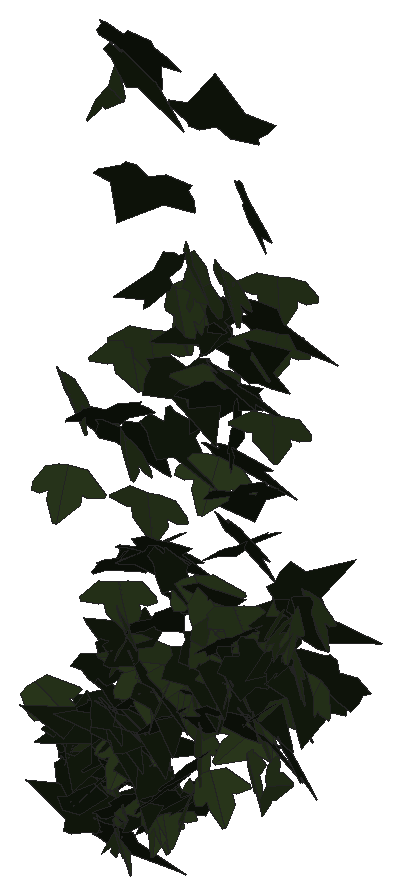
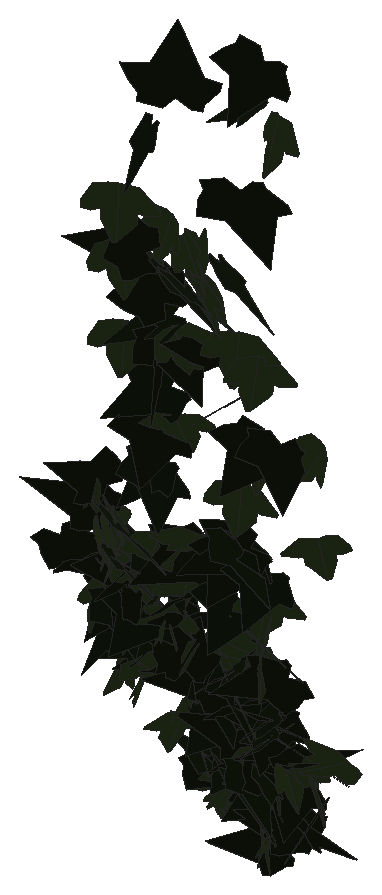
# SketchUp Ruby script. Lengths in inches.
U = 1.inch
M = Sketchup.active_model
def pt(a) = Geom::Point3d.new(a.map { |v| v * U })
def face(e, loops, mat)
  f = e.add_face(loops[0].map { |a| pt(a) })
  loops[1..].each { |l| e.add_face(l.map { |a| pt(a) }).erase! }
  f.material = f.back_material = mat if mat
  f
end
# faces: each face lists its corners as indices into pts; further lists are holes
def faces(e, pts, list, mat = nil) = list.each { |f| face(e, (f[0].is_a?(Array) ? f : [f]).map { |l| l.map { |i| pts[i] } }, mat) }
# xy, xz, yz: faces in a plane at the given z, y or x. An outline is a flat list of corners, or four numbers for a rectangle; further outlines are holes
def ring(l) = l.size == 4 ? [[l[0], l[1]], [l[2], l[1]], [l[2], l[3]], [l[0], l[3]]] : l.each_slice(2).to_a
def flat(e, list, mat, &to3) = list.each { |f| face(e, (f[0].is_a?(Array) ? f : [f]).map { |l| ring(l).map { |u, v| to3.(u, v) } }, mat) }
def xy(e, z, list, mat = nil) = flat(e, list, mat) { |x, y| [x, y, z] }
def xz(e, y, list, mat = nil) = flat(e, list, mat) { |x, z| [x, y, z] }
def yz(e, x, list, mat = nil) = flat(e, list, mat) { |y, z| [x, y, z] }
def lines(e, pts, list) = list.each { |a, b| e.add_line(pt(pts[a]), pt(pts[b])) }
# prism: a flat outline (further loops are holes) pulled along v
def prism(e, loops, v, mat = nil)
  f = face(e, loops, mat); d = Geom::Vector3d.new(v.map { |x| x * U })
  f.pushpull(f.normal.samedirection?(d) ? d.length : -d.length)
end
def box(e, o, s, mat = nil) = prism(e, [[o, [o[0] + s[0], o[1], o[2]], [o[0] + s[0], o[1] + s[1], o[2]], [o[0], o[1] + s[1], o[2]]]], [0, 0, s[2]], mat)
def at(x, y, z, deg = 0) = Geom::Transformation.translation(pt([x, y, z])) * Geom::Transformation.rotation(ORIGIN, Z_AXIS, deg.degrees)
def axes(o, x, y, z) = Geom::Transformation.new([*x, 0, *y, 0, *z, 0, *pt(o).to_a, 1])
def part(name) = M.definitions.add(name)
# library, detail: a bought-in or finely detailed component or shape, given as its bounding box
def library(name, o, s) = part(name).tap { |d| box(d.entities, o, s) }
def detail(e, o, s) = box(e.add_group.entities, o, s)
def put(e, d, t, mat = nil) = e.add_instance(d, t).tap { |i| i.material = mat if mat }
def group(e, t, mat = nil) = e.add_group.tap { |g| g.transformation = t; g.material = mat if mat }.entities
root = M.entities
M.materials.add("1026 AP 7946 SUNNY SIDE UP").color = [254, 231, 186]
M.materials.add("efeu1").color = [18, 25, 13]
M.materials.add("efeu2").color = [43, 57, 29]
c1 = part("ivyleaf_10")
p = [[0,0.5,-0.03],[-0.0625,2.02,-0.43],[-0.19,2.01,-0.46],[-0.54,1.05,-0.29],[-0.52,0.625,-0.18],[-0.83,0.76,-0.28],
  [-1.16,0.64,-0.33],[-1.15,0.33,-0.24],[-0.77,-0.39,0.02],[-0.3,-0.51,0.16],[0.04,-0.48,0.23],[-0.02,2.01,-0.4375],
  [-0.06,2.01,-0.43],[0.04,-0.49,0.23],[0.67,-0.49,0.14],[1.38,0.36,-0.2],[1.375,0.51,-0.24],[0.81,0.65,-0.19],
  [0.62,0.59,-0.15],[0.6,1.09,-0.28],[0.5,1.23,-0.31]]
faces(c1.entities,p,[[0,1,2,3,4,5,6,7,8,9,10],[11,12,0,13,14,15,16,17,18,19,20]],"efeu2")
c2 = part("ivyleaf_9")
p = [[1.54,2.16,1.25],[1.36,2.04,1.19],[-0.21,0.99,0.68],[-0.71,1.11,0.82],[-0.85,0.86,0.67],[-0.8,0.17,0.21],
  [-0.9,-0.01,0.1],[-0.67,-0.16,-0.02],[-0.08,-0.08,-0.05],[-0.03,-0.6,-0.4],[0.65,-0.88,-0.66],[0.83,-0.6,-0.49],
  [1.29,-0.42,-0.43],[1.8125,-0.07,-0.26],[1.21,0.44,0.15]]
faces(c2.entities,p,[[0,1,2,3,4,5,6,7,8,9,10,11,12,13,14]],"efeu1")
put(root,c1,axes([118.09,212.91,269.5],[0.24792,0.07326,0.21006],[0.30683,0.06038,-0.17781],[-0.14662,0.25024,-0.01692]),"1026 AP 7946 SUNNY SIDE UP")
put(root,c1,axes([118.42,212.92,272.64],[0.29256,0.20397,-0.05662],[-0.07089,-0.03479,-0.28445],[-0.325,0.1912,0.01108]),"1026 AP 7946 SUNNY SIDE UP")
put(root,c2,axes([118.43,212.86,268.69],[0.20932,-0.05573,-0.25304],[-0.25797,0.19116,-0.13534],[0.29986,0.20336,0.0602]),"1026 AP 7946 SUNNY SIDE UP")
put(root,c1,axes([118.49,212.93,269.02],[0.21124,-0.22763,0.00822],[0.0214,-0.00272,-0.2721],[0.35758,0.13463,0.01143]),"1026 AP 7946 SUNNY SIDE UP")
put(root,c1,axes([118.46,212.92,273.98],[-0.295,0.19309,-0.09552],[0.08489,-0.07815,-0.27738],[-0.3267,-0.19466,0.01417]),"1026 AP 7946 SUNNY SIDE UP")
put(root,c2,axes([118.87,212.95,269.2],[-0.11732,0.02044,0.26005],[-0.37111,-0.10071,-0.06409],[0.1439,-0.24307,0.04674]),"1026 AP 7946 SUNNY SIDE UP")
put(root,c2,axes([118.98,212.75,268.2],[-0.19293,0.10643,0.21232],[-0.26123,0.12141,-0.16626],[-0.25332,-0.20626,0.00975]),"1026 AP 7946 SUNNY SIDE UP")
put(root,c2,axes([118.83,212.96,269.2],[-0.26754,-0.19874,-0.02254],[0.04761,0.0013,-0.26856],[0.31058,-0.1714,0.02175]),"1026 AP 7946 SUNNY SIDE UP")
put(root,c2,axes([119.08,212.88,269.46],[-0.39718,0.08165,0.02283],[-0.0584,-0.04588,-0.26784],[-0.11933,-0.24934,0.05509]),"1026 AP 7946 SUNNY SIDE UP")
put(root,c1,axes([118.9,212.99,269.16],[-0.03146,-0.26053,0.00592],[-0.00776,-0.00687,-0.26918],[0.40974,-0.02013,-0.00465]),"1026 AP 7946 SUNNY SIDE UP")
put(root,c1,axes([118.8125,212.92,269.17],[0.38091,0.09128,-0.0266],[-0.02164,-0.03767,-0.26509],[-0.14782,0.24075,-0.02975]),"1026 AP 7946 SUNNY SIDE UP")
put(root,c2,axes([118.92,212.81,268.875],[0.31785,0.10905,-0.12331],[-0.17985,-0.04075,-0.23626],[-0.18124,0.23168,0.01818]),"1026 AP 7946 SUNNY SIDE UP")
put(root,c2,axes([119.09,212.88,273.84],[0.16247,0.25998,-0.05975],[-0.05027,-0.05124,-0.2883],[-0.41633,0.10764,0.0115]),"1026 AP 7946 SUNNY SIDE UP")
put(root,c2,axes([118.83,212.76,268.13],[0.11077,0.02216,0.27527],[0.41323,0.04838,-0.07526],[-0.08254,0.27194,-0.00739]),"1026 AP 7946 SUNNY SIDE UP")
put(root,c2,axes([119.18,212.98,268.8125],[0.16812,0.08963,0.22693],[-0.29764,-0.11321,0.14178],[0.22514,-0.21659,0.01797]),"1026 AP 7946 SUNNY SIDE UP")
put(root,c1,axes([119.22,212.76,278.48],[-0.04949,-0.23028,-0.236],[0.03438,0.22681,-0.23802],[0.50813,-0.03777,-0.00688]),"1026 AP 7946 SUNNY SIDE UP")
put(root,c2,axes([119.32,212.96,269.03],[-0.24075,0.12645,-0.17342],[0.14335,-0.14876,-0.20056],[-0.29942,-0.1729,0.04342]),"1026 AP 7946 SUNNY SIDE UP")
put(root,c1,axes([119.31,212.88,268.05],[0.04735,-0.25138,-0.07093],[0.00458,0.06819,-0.26019],[0.40921,0.02832,0.01112]),"1026 AP 7946 SUNNY SIDE UP")
put(root,c2,axes([119.61,212.84,269.59],[-0.30837,0.0886,0.15521],[-0.25586,-0.01186,-0.2118],[-0.09845,-0.24671,0.06429]),"1026 AP 7946 SUNNY SIDE UP")
put(root,c2,axes([119.29,212.77,269.75],[0.31651,0.16304,-0.08841],[-0.10827,-0.0528,-0.26716],[-0.26945,0.21273,0.0035]),"1026 AP 7946 SUNNY SIDE UP")
put(root,c2,axes([119.06,212.84,270.4],[0.0328,0.02519,-0.28105],[0.15959,0.25357,0.03358],[0.40038,-0.10314,0.00964]),"1026 AP 7946 SUNNY SIDE UP")
put(root,c1,axes([119.06,212.96,268.48],[0.05343,-0.00684,0.26484],[0.34112,-0.13856,-0.03414],[0.21726,0.21923,-0.01152]),"1026 AP 7946 SUNNY SIDE UP")
put(root,c2,axes([119.32,212.88,271.85],[0.18106,0.24801,0.05859],[0.04737,0.04714,-0.28132],[-0.39679,0.1188,-0.00685]),"1026 AP 7946 SUNNY SIDE UP")
put(root,c1,axes([119.3,212.87,268],[-0.12273,0.24977,-0.00755],[-0.00135,-0.00943,-0.26962],[-0.39298,-0.07797,0.00328]),"1026 AP 7946 SUNNY SIDE UP")
put(root,c1,axes([119.35,212.9,270.61],[0.05879,-0.24298,-0.1247],[0.03435,0.12311,-0.24977],[0.42449,0.02369,0.03748]),"1026 AP 7946 SUNNY SIDE UP")
put(root,c1,axes([119.4,212.82,271.06],[-0.25214,0.21535,0.07726],[-0.08709,0.05062,-0.27595],[-0.34718,-0.1691,0.01311]),"1026 AP 7946 SUNNY SIDE UP")
put(root,c2,axes([119.21,212.96,269.49],[0.04065,-0.26337,-0.00088],[-0.00091,-0.0007,-0.27263],[0.41412,0.02585,-0.00051]),"1026 AP 7946 SUNNY SIDE UP")
put(root,c2,axes([119.21,212.89,269.75],[0.07815,-0.25739,-0.06364],[-0.01244,0.0599,-0.26968],[0.41549,0.05021,0.00389]),"1026 AP 7946 SUNNY SIDE UP")
put(root,c2,axes([119.67,212.74,270.77],[-0.15701,0.19537,0.17804],[-0.20314,0.12239,-0.22013],[-0.35498,-0.15645,0.04722]),"1026 AP 7946 SUNNY SIDE UP")
put(root,c1,axes([119.37,212.8125,271.43],[-0.33033,-0.17867,-0.03595],[0.10202,-0.02528,-0.27726],[0.26713,-0.21129,0.06143]),"1026 AP 7946 SUNNY SIDE UP")
put(root,c2,axes([119.14,212.92,269.89],[0.28724,-0.19735,0.0034],[0.03742,0.01604,-0.2754],[0.30812,0.18203,0.03028]),"1026 AP 7946 SUNNY SIDE UP")
put(root,c2,axes([119.56,212.97,268.88],[-0.0665,0.25692,-0.02253],[-0.00284,-0.02393,-0.26832],[-0.40563,-0.04195,0.00557]),"1026 AP 7946 SUNNY SIDE UP")
put(root,c2,axes([119.1,212.88,267.89],[0.32602,-0.0627,0.1501],[0.22377,-0.0337,-0.22322],[0.11133,0.25137,0.0091]),"1026 AP 7946 SUNNY SIDE UP")
put(root,c1,axes([119.43,212.87,269.22],[0.2623,0.18245,-0.10579],[-0.08951,-0.0882,-0.25465],[-0.31764,0.17552,-0.0156]),"1026 AP 7946 SUNNY SIDE UP")
put(root,c2,axes([119.19,212.92,269.67],[0.29189,-0.19266,0.01676],[0.04788,0.00535,-0.27433],[0.30038,0.18636,0.02745]),"1026 AP 7946 SUNNY SIDE UP")
put(root,c1,axes([119.55,212.75,273.58],[-0.35382,0.16193,0.07425],[-0.10708,0.02695,-0.28488],[-0.25667,-0.23446,0.01649]),"1026 AP 7946 SUNNY SIDE UP")
put(root,c1,axes([119.5,212.86,274.85],[-0.31078,-0.20935,-0.03393],[0.08942,-0.01066,-0.29244],[0.32071,-0.19989,0.04867]),"1026 AP 7946 SUNNY SIDE UP")
put(root,c2,axes([119.41,212.64,268.5],[0.22845,0.15593,0.15554],[0.14414,0.11943,-0.21853],[-0.30828,0.17139,0.01309]),"1026 AP 7946 SUNNY SIDE UP")
put(root,c2,axes([119.43,212.81,273.72],[0.42519,0.10335,-0.02983],[-0.02856,-0.03489,-0.29723],[-0.16658,0.26977,-0.02518]),"1026 AP 7946 SUNNY SIDE UP")
put(root,c2,axes([119.53,212.72,279.31],[0.45636,0.04275,-0.11429],[-0.17147,-0.02247,-0.30229],[-0.07537,0.30998,-0.0043]),"1026 AP 7946 SUNNY SIDE UP")
put(root,c2,axes([119.9,212.8,268.61],[-0.18903,0.26611,0.12825],[-0.09243,0.10834,-0.30006],[-0.45159,-0.13357,0.00773]),"1026 AP 7946 SUNNY SIDE UP")
put(root,c2,axes([119.83,212.9,272.18],[-0.06925,0.27367,-0.03072],[-0.07828,-0.03916,-0.28011],[-0.42601,-0.03729,0.05647]),"1026 AP 7946 SUNNY SIDE UP")
put(root,c2,axes([119.77,212.84,277.35],[0.23768,0.16312,-0.23088],[-0.21813,-0.1777,-0.22973],[-0.3787,0.20473,-0.01258]),"1026 AP 7946 SUNNY SIDE UP")
put(root,c2,axes([119.39,212.88,278.92],[0.28834,-0.24691,-0.04076],[0.0088,0.05139,-0.3145],[0.39276,0.18012,0.03697]),"1026 AP 7946 SUNNY SIDE UP")
put(root,c1,axes([119.72,212.93,269.875],[0.1918,-0.23196,0.03149],[0.00627,-0.03389,-0.2699],[0.36811,0.12144,-0.01181]),"1026 AP 7946 SUNNY SIDE UP")
put(root,c2,axes([119.81,212.8,270.13],[0.05112,0.26282,-0.04436],[-0.00292,-0.04466,-0.27306],[-0.41915,0.03236,-0.00351]),"1026 AP 7946 SUNNY SIDE UP")
put(root,c1,axes([120.06,212.84,270.62],[0.15195,-0.01841,-0.31053],[-0.47391,0.01225,-0.10028],[0.0272,0.31621,-0.01233]),"1026 AP 7946 SUNNY SIDE UP")
put(root,c1,axes([119.82,212.87,275.11],[-0.40036,-0.14106,-0.00861],[0.02668,-0.01507,-0.29915],[0.22052,-0.25428,0.02056]),"1026 AP 7946 SUNNY SIDE UP")
put(root,c1,axes([119.84,212.81,272.85],[-0.43601,-0.05038,0.00749],[-0.00183,-0.03555,-0.28833],[0.08008,-0.27511,0.0342]),"1026 AP 7946 SUNNY SIDE UP")
put(root,c2,axes([119.71,212.9,272.04],[0.34596,0.1702,-0.01],[0.00155,-0.0187,-0.28623],[-0.26814,0.21948,-0.01456]),"1026 AP 7946 SUNNY SIDE UP")
put(root,c2,axes([119.71,212.98,269.8],[-0.05754,-0.25401,-0.06156],[0.03318,0.05581,-0.26373],[0.40845,-0.04032,0.01275]),"1026 AP 7946 SUNNY SIDE UP")
put(root,c2,axes([119.76,212.96,269],[-0.08963,-0.25246,0.03791],[-0.00522,-0.03844,-0.2668],[0.40146,-0.05687,0.00499]),"1026 AP 7946 SUNNY SIDE UP")
put(root,c1,axes([119.78,212.8,270.29],[0.34858,0.15137,0.03126],[0.01834,0.03503,-0.27539],[-0.2418,0.22088,0.02418]),"1026 AP 7946 SUNNY SIDE UP")
put(root,c2,axes([119.54,212.94,269.33],[0.15533,0.00355,0.25339],[0.37994,-0.05096,-0.09953],[0.07233,0.26009,-0.02138]),"1026 AP 7946 SUNNY SIDE UP")
put(root,c2,axes([120.13,212.77,276.11],[-0.28333,0.231,0.00236],[-0.01582,-0.0066,-0.3016],[-0.36289,-0.18007,0.0113]),"1026 AP 7946 SUNNY SIDE UP")
put(root,c2,axes([119.66,212.85,272.125],[0.38923,0.08284,0.10481],[0.1509,0.03233,-0.26872],[-0.13982,0.26549,0.00175]),"1026 AP 7946 SUNNY SIDE UP")
put(root,c2,axes([119.9,212.79,271.23],[0.19588,0.23998,0.07547],[0.05909,0.06148,-0.27814],[-0.38945,0.13003,-0.00425]),"1026 AP 7946 SUNNY SIDE UP")
put(root,c2,axes([119.71,212.89,270.46],[0.2171,-0.23327,0.02932],[0.02259,-0.02611,-0.27941],[0.36909,0.13881,-0.00014]),"1026 AP 7946 SUNNY SIDE UP")
put(root,c1,axes([119.92,212.87,268.5],[0.08163,0.232,-0.11757],[-0.02611,-0.11452,-0.24545],[-0.40663,0.05393,-0.00784]),"1026 AP 7946 SUNNY SIDE UP")
put(root,c1,axes([119.91,212.875,268.52],[0.05957,0.26157,0.00913],[0.00215,0.00726,-0.27224],[-0.41145,0.03791,-0.0001]),"1026 AP 7946 SUNNY SIDE UP")
put(root,c1,axes([119.96,212.9,270.19],[0.19196,-0.22935,0.069],[0.0426,-0.06292,-0.26797],[0.37385,0.12493,-0.0049]),"1026 AP 7946 SUNNY SIDE UP")
put(root,c1,axes([119.98,212.87,268.59],[-0.33521,-0.15583,-0.01871],[0.08969,-0.04992,-0.26149],[0.22964,-0.20797,0.07482]),"1026 AP 7946 SUNNY SIDE UP")
put(root,c2,axes([120.04,212.61,268.83],[0.11542,0.20422,0.15552],[0.07352,0.14235,-0.2227],[-0.39139,0.08697,0.00403]),"1026 AP 7946 SUNNY SIDE UP")
put(root,c2,axes([120.15,212.82,269.93],[0.02019,0.26238,-0.04788],[0.00618,-0.04821,-0.27084],[-0.41937,0.01192,-0.0063]),"1026 AP 7946 SUNNY SIDE UP")
put(root,c2,axes([119.95,212.97,270.16],[-0.02898,-0.26674,0.01718],[0.00756,-0.01856,-0.27549],[0.42033,-0.01806,0.00614]),"1026 AP 7946 SUNNY SIDE UP")
put(root,c2,axes([120.25,212.87,268.79],[0.01472,0.18553,-0.19465],[-0.05826,-0.18735,-0.19144],[-0.41349,0.033,0.02004]),"1026 AP 7946 SUNNY SIDE UP")
put(root,c1,axes([120.5,212.94,270.06],[-0.19425,-0.01762,0.30213],[-0.4318,-0.1065,-0.12634],[0.1647,-0.29999,0.02512]),"1026 AP 7946 SUNNY SIDE UP")
put(root,c1,axes([120.23,212.91,270.47],[-0.30344,-0.18895,0.02803],[0.0458,-0.06882,-0.26935],[0.2969,-0.18249,0.0702]),"1026 AP 7946 SUNNY SIDE UP")
put(root,c2,axes([120.11,212.78,272.17],[0.20957,-0.22413,-0.11483],[-0.10223,0.08946,-0.26794],[0.37917,0.14799,-0.00877]),"1026 AP 7946 SUNNY SIDE UP")
put(root,c2,axes([120.49,212.87,268.94],[-0.24812,0.20125,-0.0764],[-0.00053,-0.09366,-0.25769],[-0.33788,-0.14764,0.05651]),"1026 AP 7946 SUNNY SIDE UP")
put(root,c2,axes([119.97,213,270.05],[0.31919,-0.02021,0.1755],[0.26992,0.02485,-0.20741],[-0.00098,0.26391,0.03454]),"1026 AP 7946 SUNNY SIDE UP")
put(root,c1,axes([120.26,212.9,275.78],[-0.35801,0.13822,-0.12504],[0.06818,-0.14851,-0.25724],[-0.28192,-0.21144,0.09657]),"1026 AP 7946 SUNNY SIDE UP")
put(root,c2,axes([120.11,212.79,274.04],[0.18543,-0.24109,-0.11764],[0.00481,0.12462,-0.27031],[0.41852,0.10539,0.05523]),"1026 AP 7946 SUNNY SIDE UP")
put(root,c1,axes([120.38,212.875,268.86],[0.15396,-0.24549,-0.0346],[0.00094,0.03485,-0.27172],[0.38931,0.097,0.01434]),"1026 AP 7946 SUNNY SIDE UP")
put(root,c1,axes([120.4,212.93,275.82],[0.34755,-0.1884,-0.04956],[-0.05419,0.03207,-0.29901],[0.30049,0.22369,0.0034]),"1026 AP 7946 SUNNY SIDE UP")
put(root,c1,axes([120.31,212.93,270.375],[0.41542,-0.03348,0.00795],[0.01806,0.02813,-0.27252],[0.05099,0.26281,0.03176]),"1026 AP 7946 SUNNY SIDE UP")
put(root,c2,axes([120.375,212.64,269.24],[0.10668,0.18774,0.17985],[0.09687,0.16223,-0.20468],[-0.39013,0.09162,-0.00164]),"1026 AP 7946 SUNNY SIDE UP")
put(root,c1,axes([120.43,212.98,270.41],[-0.07147,0.25268,-0.07748],[0.00037,-0.07773,-0.26461],[-0.41519,-0.04357,0.0131]),"1026 AP 7946 SUNNY SIDE UP")
put(root,c1,axes([120.75,212.81,276.2],[-0.25395,0.11277,0.23126],[-0.33293,0.08111,-0.199],[-0.2109,-0.26383,0.03569]),"1026 AP 7946 SUNNY SIDE UP")
put(root,c2,axes([120.43,213.18,270.24],[0.41647,-0.17045,0.05057],[-0.03338,0.05885,0.32251],[-0.27733,-0.26305,0.03712]),"1026 AP 7946 SUNNY SIDE UP")
put(root,c2,axes([120.39,212.85,274.86],[-0.17008,-0.2038,-0.18947],[0.14621,0.15747,-0.23667],[0.40483,-0.14249,0.00588]),"1026 AP 7946 SUNNY SIDE UP")
put(root,c1,axes([120.3,212.97,276.15],[-0.05024,0.03649,0.33534],[0.41387,-0.19146,0.04764],[0.30602,0.26493,-0.00938]),"1026 AP 7946 SUNNY SIDE UP")
put(root,c1,axes([120.55,212.96,269.69],[-0.01948,0.23876,-0.11822],[-0.0135,-0.11654,-0.24661],[-0.41726,-0.00738,0.0135]),"1026 AP 7946 SUNNY SIDE UP")
put(root,c2,axes([120.9,212.86,275.72],[-0.37522,0.17194,0.00267],[-0.04796,-0.03961,-0.29883],[-0.26608,-0.23532,0.0501]),"1026 AP 7946 SUNNY SIDE UP")
put(root,c1,axes([120.78,212.9,274.88],[-0.25488,-0.21637,0.11244],[-0.03778,-0.11776,-0.27486],[0.38005,-0.15681,0.04808]),"1026 AP 7946 SUNNY SIDE UP")
put(root,c1,axes([120.86,212.85,270.67],[0.25222,-0.14246,-0.20969],[-0.21501,0.15051,-0.21953],[0.32491,0.21019,0.0175]),"1026 AP 7946 SUNNY SIDE UP")
put(root,c2,axes([120.61,212.9375,270.8],[-0.14965,-0.23164,-0.11078],[0.07998,0.09384,-0.25721],[0.39263,-0.1074,0.01017]),"1026 AP 7946 SUNNY SIDE UP")
put(root,c2,axes([120.47,212.81,271.74],[0.42263,0.08777,0.08904],[0.14219,-0.00148,-0.28984],[-0.13071,0.28218,-0.0274]),"1026 AP 7946 SUNNY SIDE UP")
put(root,c1,axes([120.6,212.81,271.89],[0.32652,0.16496,0.10255],[0.07776,0.09443,-0.26946],[-0.29202,0.20959,0.04292]),"1026 AP 7946 SUNNY SIDE UP")
put(root,c2,axes([121.03,212.8,275.73],[-0.28656,0.23084,0.02911],[-0.05684,0.00567,-0.30188],[-0.36099,-0.18414,0.02443]),"1026 AP 7946 SUNNY SIDE UP")
put(root,c1,axes([120.76,212.78,271.19],[0.1252,0.25872,0.04486],[-0.05361,0.05383,-0.27416],[-0.40865,0.0722,0.04971]),"1026 AP 7946 SUNNY SIDE UP")
put(root,c1,axes([120.75,212.6,271.6],[0.02684,-0.00644,-0.3148],[0.12568,0.29546,-0.00009],[0.46381,-0.07969,0.01824]),"1026 AP 7946 SUNNY SIDE UP")
put(root,c2,axes([120.96,212.83,274.79],[0.10966,0.21288,-0.19543],[-0.07829,-0.18447,-0.23172],[-0.44275,0.08534,-0.00743]),"1026 AP 7946 SUNNY SIDE UP")
put(root,c2,axes([120.71,212.92,271.04],[-0.00221,-0.2737,-0.01387],[-0.0048,0.01193,-0.28188],[0.43075,-0.00127,-0.00321]),"1026 AP 7946 SUNNY SIDE UP")
put(root,c1,axes([120.81,212.86,273.63],[0.3845,0.13749,-0.05598],[-0.04828,-0.05704,-0.28721],[-0.22787,0.24409,-0.03362]),"1026 AP 7946 SUNNY SIDE UP")
put(root,c1,axes([120.79,212.87,269.2],[0.1532,0.24869,0.02156],[0.01117,0.01818,-0.27505],[-0.39208,0.09769,0.00059]),"1026 AP 7946 SUNNY SIDE UP")
put(root,c2,axes([120.84,212.87,278.47],[0.45063,0.01874,0.14921],[-0.22947,0.03799,0.29286],[-0.00085,-0.3188,0.04177]),"1026 AP 7946 SUNNY SIDE UP")
put(root,c1,axes([120.97,212.84,270.52],[0.19446,-0.23796,-0.03966],[0.01678,0.04713,-0.27416],[0.37833,0.12022,0.03255]),"1026 AP 7946 SUNNY SIDE UP")
put(root,c2,axes([120.76,212.74,270.16],[0.37727,0.05257,0.1222],[0.17961,0.03135,-0.25279],[-0.09584,0.26568,0.00729]),"1026 AP 7946 SUNNY SIDE UP")
put(root,c1,axes([120.8,212.89,270.67],[-0.16595,-0.09318,-0.23743],[0.35505,0.06748,-0.13454],[0.16167,-0.24384,0.05176]),"1026 AP 7946 SUNNY SIDE UP")
put(root,c2,axes([121.18,212.77,274.42],[0.06942,-0.03546,-0.32808],[-0.4023,0.18931,-0.05718],[0.30282,0.25962,-0.00076]),"1026 AP 7946 SUNNY SIDE UP")
put(root,c1,axes([121.07,212.93,270.67],[-0.26169,0.21009,-0.01226],[-0.01343,-0.02342,-0.27539],[-0.33071,-0.16529,0.02089]),"1026 AP 7946 SUNNY SIDE UP")
put(root,c2,axes([121.22,212.7,271.47],[-0.00566,0.26887,-0.06067],[-0.03487,-0.06051,-0.2764],[-0.43191,0.00136,0.02311]),"1026 AP 7946 SUNNY SIDE UP")
put(root,c1,axes([121.08,212.77,276.42],[-0.36083,0.18735,-0.00897],[-0.01246,-0.02511,-0.3043],[-0.29473,-0.22831,0.02385]),"1026 AP 7946 SUNNY SIDE UP")
put(root,c2,axes([121.22,212.8,272.72],[0.08905,0.2782,0.0274],[-0.02846,0.02913,-0.29131],[-0.43829,0.05463,0.02448]),"1026 AP 7946 SUNNY SIDE UP")
put(root,c1,axes([121.21,213.08,269.97],[0.25755,0.11467,-0.18007],[-0.19495,-0.12651,-0.20517],[-0.26571,0.20397,-0.024]),"1026 AP 7946 SUNNY SIDE UP")
put(root,c2,axes([121.14,212.84,273.42],[0.23959,0.24177,-0.01432],[0.00435,-0.01978,-0.29422],[-0.38089,0.15185,-0.01237]),"1026 AP 7946 SUNNY SIDE UP")
put(root,c2,axes([121.02,212.86,271.16],[0.25136,-0.18121,-0.13215],[-0.13664,0.09301,-0.24837],[0.32023,0.18192,-0.00225]),"1026 AP 7946 SUNNY SIDE UP")
put(root,c1,axes([121.16,212.88,271.68],[-0.34464,-0.16079,-0.06312],[0.12341,-0.00672,-0.27519],[0.24021,-0.22724,0.05081]),"1026 AP 7946 SUNNY SIDE UP")
put(root,c2,axes([121.59,212.92,271.22],[-0.27281,0.1686,0.12454],[-0.23237,0.00857,-0.2326],[-0.22771,-0.21074,0.08815]),"1026 AP 7946 SUNNY SIDE UP")
put(root,c2,axes([121.1,212.85,272.9],[0.41899,-0.07315,-0.07681],[-0.11859,0.00495,-0.28424],[0.11295,0.27655,-0.0135]),"1026 AP 7946 SUNNY SIDE UP")
put(root,c1,axes([121.41,212.97,271.31],[-0.37627,-0.08777,0.09506],[-0.10869,-0.07667,-0.25885],[0.16886,-0.24493,0.0452]),"1026 AP 7946 SUNNY SIDE UP")
put(root,c2,axes([121.04,212.74,275.06],[0.42137,-0.10974,-0.04737],[-0.01477,0.09201,-0.28599],[0.18613,0.25574,0.08454]),"1026 AP 7946 SUNNY SIDE UP")
put(root,c2,axes([121.05,212.77,273.99],[0.44944,-0.00937,0.02965],[0.04631,0.02072,-0.29366],[0.01136,0.28653,0.02389]),"1026 AP 7946 SUNNY SIDE UP")
put(root,c2,axes([121.21,212.91,270.68],[0.34821,0.15081,0.02603],[-0.00012,0.0431,-0.27333],[-0.24023,0.21858,0.03787]),"1026 AP 7946 SUNNY SIDE UP")
put(root,c1,axes([121.39,212.87,269.65],[-0.12184,0.25718,-0.02761],[-0.00206,-0.02989,-0.2767],[-0.40682,-0.07687,0.00967]),"1026 AP 7946 SUNNY SIDE UP")
put(root,c2,axes([121.09,212.85,275.32],[0.49078,-0.02004,-0.11167],[0.173,0.07101,0.31356],[0.00759,-0.32265,0.07396]),"1026 AP 7946 SUNNY SIDE UP")
put(root,c2,axes([121.44,212.67,277.65],[0.2853,-0.06505,-0.23976],[-0.31545,0.12088,-0.19554],[0.21083,0.26889,0.03189]),"1026 AP 7946 SUNNY SIDE UP")
put(root,c2,axes([121.35,212.72,271.23],[0.13762,-0.09335,-0.25256],[-0.06121,0.25042,-0.11133],[0.40713,0.06921,0.06863]),"1026 AP 7946 SUNNY SIDE UP")
put(root,c1,axes([121.47,212.93,270.36],[-0.06918,0.26636,-0.01108],[0.00016,-0.01241,-0.27818],[-0.41926,-0.04396,0.00172]),"1026 AP 7946 SUNNY SIDE UP")
put(root,c2,axes([121.29,212.95,270.25],[0.31393,-0.17926,0.00519],[0.01057,-0.00157,-0.27641],[0.28184,0.19974,0.00459]),"1026 AP 7946 SUNNY SIDE UP")
put(root,c2,axes([121.85,212.93,271.89],[-0.25309,0.21406,0.07308],[-0.10948,0.03417,-0.27348],[-0.33663,-0.17205,0.034]),"1026 AP 7946 SUNNY SIDE UP")
put(root,c2,axes([121.36,212.86,270.79],[-0.10901,-0.0979,-0.2522],[0.36628,0.09465,-0.10665],[0.19245,-0.2356,0.06012]),"1026 AP 7946 SUNNY SIDE UP")
put(root,c2,axes([121.8,212.93,270.64],[-0.04625,0.26122,-0.06876],[0.0002,-0.06862,-0.27111],[-0.42453,-0.02849,0.00736]),"1026 AP 7946 SUNNY SIDE UP")
put(root,c2,axes([121.9,212.92,271.39],[-0.29389,0.1971,0.0037],[-0.02913,-0.01417,-0.27889],[-0.30858,-0.18638,0.0228]),"1026 AP 7946 SUNNY SIDE UP")
put(root,c1,axes([121.75,212.84,274.6],[-0.39638,-0.14332,0.00472],[0.00833,-0.0202,-0.29813],[0.22536,-0.25133,0.01931]),"1026 AP 7946 SUNNY SIDE UP")
put(root,c1,axes([121.79,212.84,275.77],[-0.36518,-0.18284,0.03555],[-0.02262,-0.03903,-0.30391],[0.292,-0.23168,0.02091]),"1026 AP 7946 SUNNY SIDE UP")
put(root,c1,axes([121.75,212.93,271.87],[0.14241,-0.26231,0.00434],[0.00187,-0.00562,-0.28592],[0.41255,0.09058,-0.0002]),"1026 AP 7946 SUNNY SIDE UP")
put(root,c2,axes([121.37,212.89,275.95],[0.33413,-0.07183,0.20227],[0.27202,-0.09782,-0.22984],[0.18568,0.27257,-0.02727]),"1026 AP 7946 SUNNY SIDE UP")
put(root,c2,axes([121.64,212.95,270.87],[0.43705,-0.04875,-0.09945],[-0.15556,-0.00895,-0.28966],[0.06773,0.29401,-0.02354]),"1026 AP 7946 SUNNY SIDE UP")
put(root,c1,axes([121.77,212.98,271.4375],[-0.21562,0.23611,-0.00416],[-0.00938,-0.00968,-0.28115],[-0.37123,-0.13689,0.00952]),"1026 AP 7946 SUNNY SIDE UP")
put(root,c1,axes([121.85,212.82,276.59],[-0.41441,-0.14374,0.00042],[0.01139,-0.01582,-0.30884],[0.22574,-0.26308,0.01635]),"1026 AP 7946 SUNNY SIDE UP")
put(root,c1,axes([121.82,212.66,269.63],[0.01019,-0.13354,-0.26416],[0.0712,0.25302,-0.13349],[0.44791,-0.03718,0.02723]),"1026 AP 7946 SUNNY SIDE UP")
put(root,c1,axes([121.9,212.92,271.8],[0.05292,-0.27538,0.00836],[0.00024,-0.00974,-0.28586],[0.43327,0.03364,-0.00086]),"1026 AP 7946 SUNNY SIDE UP")
put(root,c1,axes([121.98,212.99,271.67],[0.07574,-0.26921,0.00461],[-0.00023,-0.00612,-0.28177],[0.4234,0.04815,-0.00098]),"1026 AP 7946 SUNNY SIDE UP")
put(root,c1,axes([121.95,212.92,270.71],[-0.21831,-0.21046,-0.10739],[0.0983,0.08216,-0.25918],[0.3551,-0.15213,0.00573]),"1026 AP 7946 SUNNY SIDE UP")
put(root,c2,axes([121.92,212.82,270.17],[0.30915,-0.13034,-0.1407],[-0.19098,0.06224,-0.24227],[0.22616,0.23072,-0.01225]),"1026 AP 7946 SUNNY SIDE UP")
put(root,c1,axes([121.91,212.9,271.94],[0.34277,-0.14268,0.10279],[0.13973,-0.04782,-0.26856],[0.23628,0.23527,0.00969]),"1026 AP 7946 SUNNY SIDE UP")
put(root,c1,axes([122.03,212.87,271.43],[-0.21457,0.21669,-0.09558],[0.04836,-0.09135,-0.26344],[-0.36825,-0.13826,0.0211]),"1026 AP 7946 SUNNY SIDE UP")
put(root,c2,axes([122.03,212.85,272.26],[-0.01259,0.01641,0.28734],[0.37268,0.14797,-0.0011],[-0.23235,0.23645,-0.01733]),"1026 AP 7946 SUNNY SIDE UP")
put(root,c1,axes([122.27,212.91,272.25],[-0.33068,0.1626,-0.08431],[0.08031,-0.06878,-0.27331],[-0.27542,-0.21528,0.02154]),"1026 AP 7946 SUNNY SIDE UP")
put(root,c2,axes([122.6,213,271.32],[0.04529,0.05822,-0.27321],[-0.31511,-0.17587,-0.06315],[-0.28882,0.20101,0.02606]),"1026 AP 7946 SUNNY SIDE UP")
put(root,c2,axes([122.29,212.95,271.08],[-0.16529,-0.25099,0.0127],[0.00349,-0.01584,-0.2803],[0.39524,-0.10482,0.00779]),"1026 AP 7946 SUNNY SIDE UP")
put(root,c1,axes([122.35,212.86,271.0625],[0.37114,-0.13573,-0.0189],[-0.03699,-0.00572,-0.28001],[0.212,0.23662,-0.01577]),"1026 AP 7946 SUNNY SIDE UP")
put(root,c2,axes([122.04,212.93,271.89],[0.19157,-0.02065,0.25602],[0.36292,-0.09573,-0.12526],[0.14895,0.2598,-0.02408]),"1026 AP 7946 SUNNY SIDE UP")
